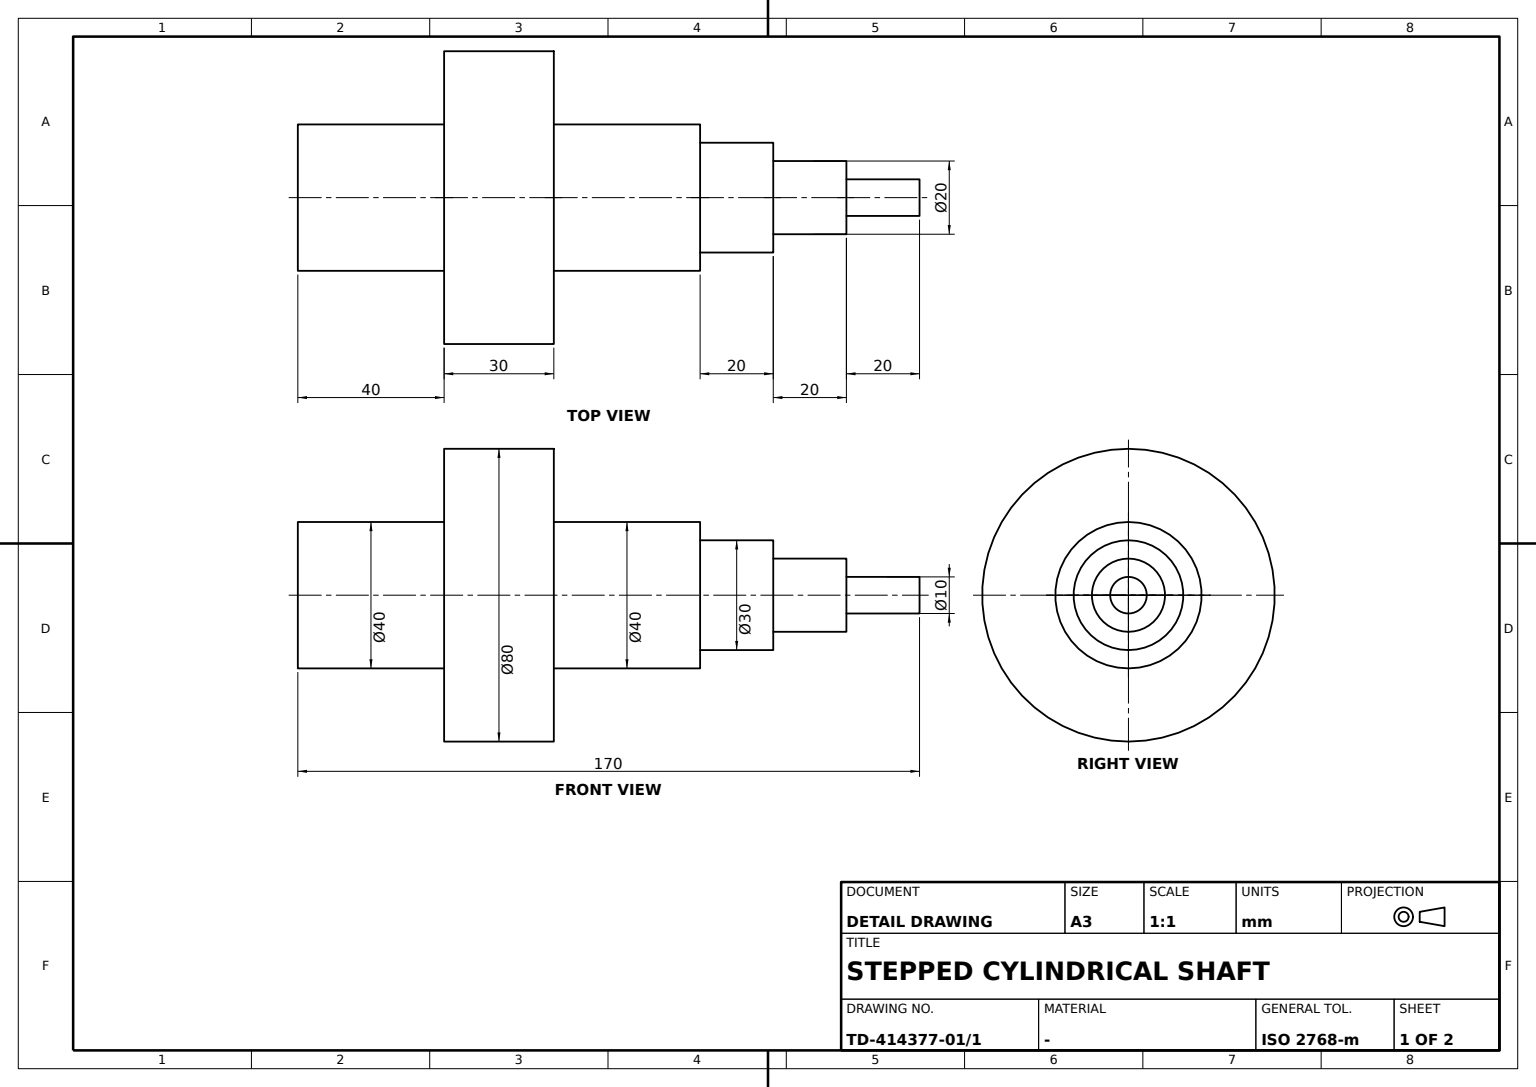
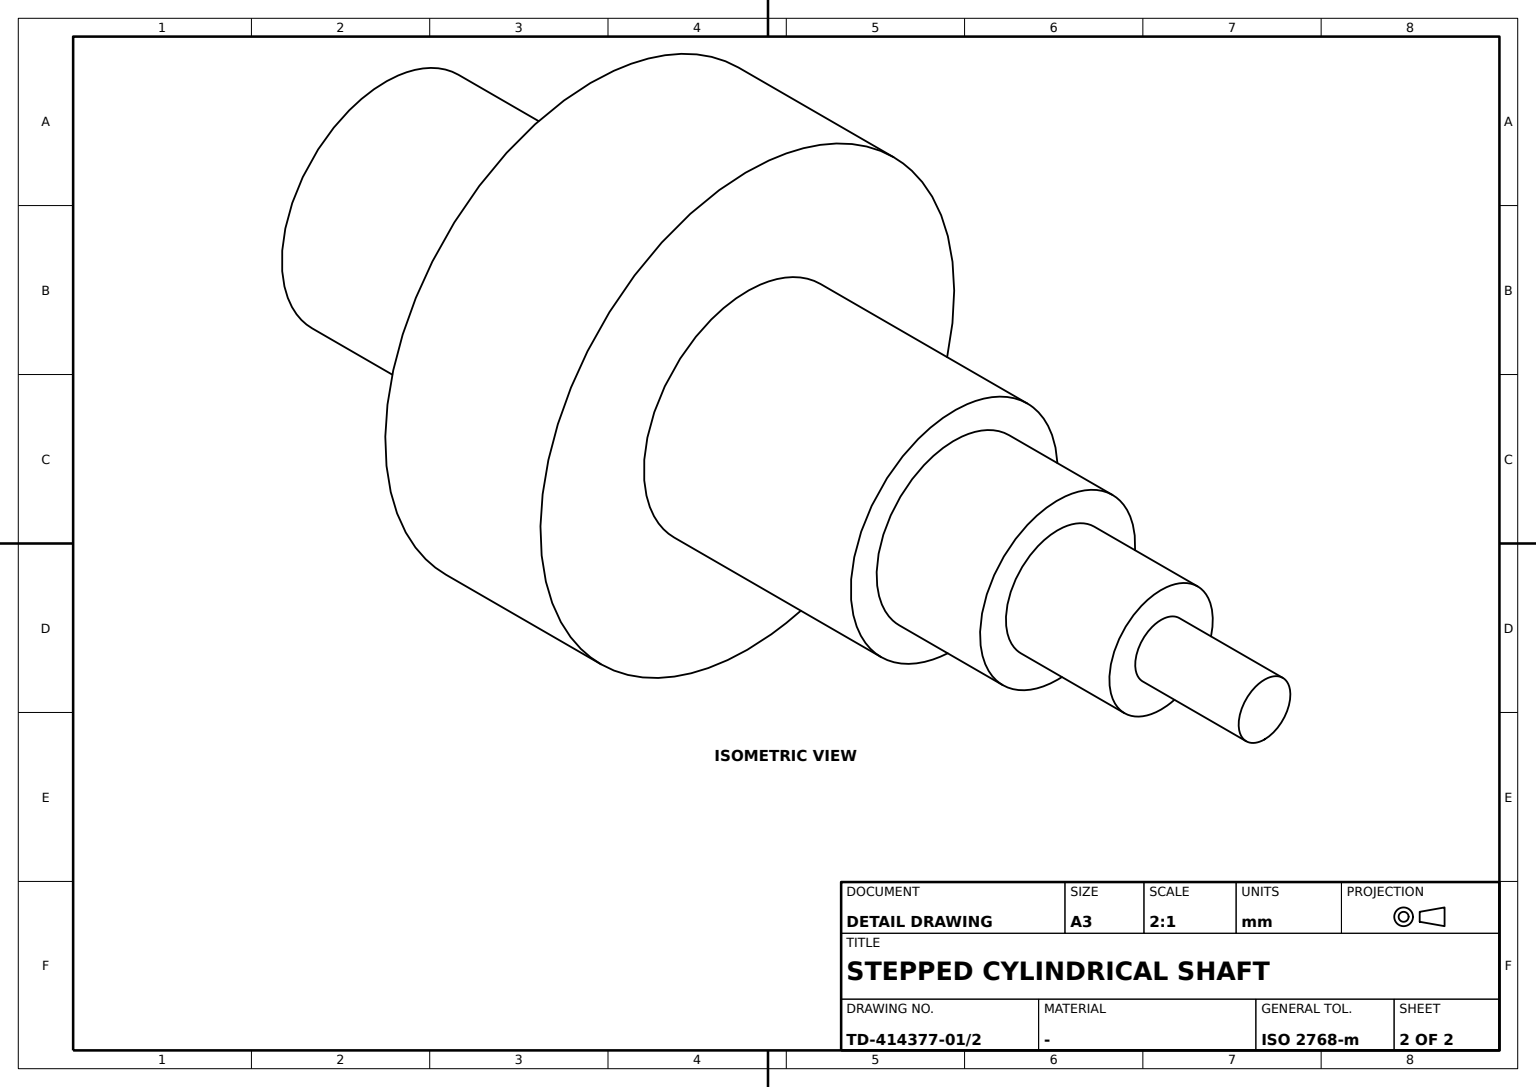
ISO-10303-21;
HEADER;
FILE_DESCRIPTION((''),'2;1');
FILE_NAME('','',(''),(''),'','','');
FILE_SCHEMA(('AUTOMOTIVE_DESIGN'));
ENDSEC;
DATA;
#1=APPLICATION_CONTEXT('');
#2=PRODUCT_CONTEXT('',#1,'mechanical');
#3=PRODUCT('','','',(#2));
#4=PRODUCT_DEFINITION_FORMATION('','',#3);
#5=PRODUCT_DEFINITION_CONTEXT('',#1,'design');
#6=PRODUCT_DEFINITION('','',#4,#5);
#7=PRODUCT_DEFINITION_SHAPE('','',#6);
#8=(LENGTH_UNIT()NAMED_UNIT(*)SI_UNIT(.MILLI.,.METRE.));
#9=(NAMED_UNIT(*)PLANE_ANGLE_UNIT()SI_UNIT($,.RADIAN.));
#10=(NAMED_UNIT(*)SI_UNIT($,.STERADIAN.)SOLID_ANGLE_UNIT());
#11=UNCERTAINTY_MEASURE_WITH_UNIT(LENGTH_MEASURE(0.005),#8,'distance_accuracy_value','');
#12=(GEOMETRIC_REPRESENTATION_CONTEXT(3)GLOBAL_UNCERTAINTY_ASSIGNED_CONTEXT((#11))GLOBAL_UNIT_ASSIGNED_CONTEXT((#8,#9,#10))REPRESENTATION_CONTEXT('',''));
#13=CARTESIAN_POINT('',(-42.006329,0.,-20.));
#14=VERTEX_POINT('',#13);
#15=CARTESIAN_POINT('',(-42.006329,0.,0.));
#16=DIRECTION('',(1.,0.,0.));
#17=DIRECTION('',(0.,0.,-1.));
#18=AXIS2_PLACEMENT_3D('',#15,#16,#17);
#19=CIRCLE('',#18,20.);
#20=EDGE_CURVE('',#14,#14,#19,.T.);
#21=ORIENTED_EDGE('',*,*,#20,.F.);
#22=EDGE_LOOP('',(#21));
#23=FACE_BOUND('',#22,.T.);
#24=CARTESIAN_POINT('',(-42.006329,0.,-40.));
#25=VERTEX_POINT('',#24);
#26=CIRCLE('',#18,40.);
#27=EDGE_CURVE('',#25,#25,#26,.T.);
#28=ORIENTED_EDGE('',*,*,#27,.T.);
#29=EDGE_LOOP('',(#28));
#30=FACE_BOUND('',#29,.T.);
#31=CARTESIAN_POINT('',(-42.006329,-40.,0.));
#32=DIRECTION('',(0.,1.,0.));
#33=AXIS2_PLACEMENT_3D('',#31,#16,#32);
#34=PLANE('',#33);
#35=ADVANCED_FACE('',(#23,#30),#34,.T.);
#36=CARTESIAN_POINT('',(-72.006329,0.,-20.));
#37=VERTEX_POINT('',#36);
#38=CARTESIAN_POINT('',(-72.006329,0.,0.));
#39=AXIS2_PLACEMENT_3D('',#38,#16,#17);
#40=CIRCLE('',#39,20.);
#41=EDGE_CURVE('',#37,#37,#40,.T.);
#42=ORIENTED_EDGE('',*,*,#41,.T.);
#43=EDGE_LOOP('',(#42));
#44=FACE_BOUND('',#43,.T.);
#45=CARTESIAN_POINT('',(-72.006329,0.,-40.));
#46=VERTEX_POINT('',#45);
#47=CIRCLE('',#39,40.);
#48=EDGE_CURVE('',#46,#46,#47,.T.);
#49=ORIENTED_EDGE('',*,*,#48,.F.);
#50=EDGE_LOOP('',(#49));
#51=FACE_BOUND('',#50,.T.);
#52=CARTESIAN_POINT('',(-72.006329,-20.,0.));
#53=AXIS2_PLACEMENT_3D('',#52,#16,#32);
#54=PLANE('',#53);
#55=ADVANCED_FACE('',(#44,#51),#54,.F.);
#56=CARTESIAN_POINT('',(17.993671,0.,-10.));
#57=VERTEX_POINT('',#56);
#58=CARTESIAN_POINT('',(17.993671,0.,0.));
#59=AXIS2_PLACEMENT_3D('',#58,#16,#17);
#60=CIRCLE('',#59,10.);
#61=EDGE_CURVE('',#57,#57,#60,.T.);
#62=ORIENTED_EDGE('',*,*,#61,.F.);
#63=EDGE_LOOP('',(#62));
#64=FACE_BOUND('',#63,.T.);
#65=CARTESIAN_POINT('',(17.993671,0.,-15.));
#66=VERTEX_POINT('',#65);
#67=CIRCLE('',#59,15.);
#68=EDGE_CURVE('',#66,#66,#67,.T.);
#69=ORIENTED_EDGE('',*,*,#68,.T.);
#70=EDGE_LOOP('',(#69));
#71=FACE_BOUND('',#70,.T.);
#72=CARTESIAN_POINT('',(17.993671,-15.,0.));
#73=AXIS2_PLACEMENT_3D('',#72,#16,#32);
#74=PLANE('',#73);
#75=ADVANCED_FACE('',(#64,#71),#74,.T.);
#76=ORIENTED_EDGE('',*,*,#41,.F.);
#77=EDGE_LOOP('',(#76));
#78=FACE_BOUND('',#77,.T.);
#79=CARTESIAN_POINT('',(-112.006329,0.,-20.));
#80=VERTEX_POINT('',#79);
#81=CARTESIAN_POINT('',(-112.006329,0.,0.));
#82=AXIS2_PLACEMENT_3D('',#81,#16,#17);
#83=CIRCLE('',#82,20.);
#84=EDGE_CURVE('',#80,#80,#83,.T.);
#85=ORIENTED_EDGE('',*,*,#84,.T.);
#86=EDGE_LOOP('',(#85));
#87=FACE_BOUND('',#86,.T.);
#88=CARTESIAN_POINT('',(-27.006329,0.,0.));
#89=AXIS2_PLACEMENT_3D('',#88,#16,#32);
#90=CYLINDRICAL_SURFACE('',#89,20.);
#91=ADVANCED_FACE('',(#78,#87),#90,.T.);
#92=CARTESIAN_POINT('',(57.993671,0.,-5.));
#93=VERTEX_POINT('',#92);
#94=CARTESIAN_POINT('',(57.993671,0.,0.));
#95=AXIS2_PLACEMENT_3D('',#94,#16,#17);
#96=CIRCLE('',#95,5.);
#97=EDGE_CURVE('',#93,#93,#96,.T.);
#98=ORIENTED_EDGE('',*,*,#97,.F.);
#99=EDGE_LOOP('',(#98));
#100=FACE_BOUND('',#99,.T.);
#101=CARTESIAN_POINT('',(37.993671,0.,-5.));
#102=VERTEX_POINT('',#101);
#103=CARTESIAN_POINT('',(37.993671,0.,0.));
#104=AXIS2_PLACEMENT_3D('',#103,#16,#17);
#105=CIRCLE('',#104,5.);
#106=EDGE_CURVE('',#102,#102,#105,.T.);
#107=ORIENTED_EDGE('',*,*,#106,.T.);
#108=EDGE_LOOP('',(#107));
#109=FACE_BOUND('',#108,.T.);
#110=CYLINDRICAL_SURFACE('',#89,5.);
#111=ADVANCED_FACE('',(#100,#109),#110,.T.);
#112=ORIENTED_EDGE('',*,*,#84,.F.);
#113=EDGE_LOOP('',(#112));
#114=FACE_BOUND('',#113,.T.);
#115=AXIS2_PLACEMENT_3D('',#81,#16,#32);
#116=PLANE('',#115);
#117=ADVANCED_FACE('',(#114),#116,.F.);
#118=ORIENTED_EDGE('',*,*,#97,.T.);
#119=EDGE_LOOP('',(#118));
#120=FACE_BOUND('',#119,.T.);
#121=CARTESIAN_POINT('',(57.993671,-5.,0.));
#122=AXIS2_PLACEMENT_3D('',#121,#16,#32);
#123=PLANE('',#122);
#124=ADVANCED_FACE('',(#120),#123,.T.);
#125=ORIENTED_EDGE('',*,*,#68,.F.);
#126=EDGE_LOOP('',(#125));
#127=FACE_BOUND('',#126,.T.);
#128=CARTESIAN_POINT('',(-2.006329,0.,-15.));
#129=VERTEX_POINT('',#128);
#130=CARTESIAN_POINT('',(-2.006329,0.,0.));
#131=AXIS2_PLACEMENT_3D('',#130,#16,#17);
#132=CIRCLE('',#131,15.);
#133=EDGE_CURVE('',#129,#129,#132,.T.);
#134=ORIENTED_EDGE('',*,*,#133,.T.);
#135=EDGE_LOOP('',(#134));
#136=FACE_BOUND('',#135,.T.);
#137=CYLINDRICAL_SURFACE('',#89,15.);
#138=ADVANCED_FACE('',(#127,#136),#137,.T.);
#139=CARTESIAN_POINT('',(-2.006329,0.,-20.));
#140=VERTEX_POINT('',#139);
#141=CIRCLE('',#131,20.);
#142=EDGE_CURVE('',#140,#140,#141,.T.);
#143=ORIENTED_EDGE('',*,*,#142,.F.);
#144=EDGE_LOOP('',(#143));
#145=FACE_BOUND('',#144,.T.);
#146=ORIENTED_EDGE('',*,*,#20,.T.);
#147=EDGE_LOOP('',(#146));
#148=FACE_BOUND('',#147,.T.);
#149=ADVANCED_FACE('',(#145,#148),#90,.T.);
#150=ORIENTED_EDGE('',*,*,#106,.F.);
#151=EDGE_LOOP('',(#150));
#152=FACE_BOUND('',#151,.T.);
#153=CARTESIAN_POINT('',(37.993671,0.,-10.));
#154=VERTEX_POINT('',#153);
#155=CIRCLE('',#104,10.);
#156=EDGE_CURVE('',#154,#154,#155,.T.);
#157=ORIENTED_EDGE('',*,*,#156,.T.);
#158=EDGE_LOOP('',(#157));
#159=FACE_BOUND('',#158,.T.);
#160=CARTESIAN_POINT('',(37.993671,-10.,0.));
#161=AXIS2_PLACEMENT_3D('',#160,#16,#32);
#162=PLANE('',#161);
#163=ADVANCED_FACE('',(#152,#159),#162,.T.);
#164=ORIENTED_EDGE('',*,*,#133,.F.);
#165=EDGE_LOOP('',(#164));
#166=FACE_BOUND('',#165,.T.);
#167=ORIENTED_EDGE('',*,*,#142,.T.);
#168=EDGE_LOOP('',(#167));
#169=FACE_BOUND('',#168,.T.);
#170=CARTESIAN_POINT('',(-2.006329,-20.,0.));
#171=AXIS2_PLACEMENT_3D('',#170,#16,#32);
#172=PLANE('',#171);
#173=ADVANCED_FACE('',(#166,#169),#172,.T.);
#174=ORIENTED_EDGE('',*,*,#48,.T.);
#175=EDGE_LOOP('',(#174));
#176=FACE_BOUND('',#175,.T.);
#177=ORIENTED_EDGE('',*,*,#27,.F.);
#178=EDGE_LOOP('',(#177));
#179=FACE_BOUND('',#178,.T.);
#180=CYLINDRICAL_SURFACE('',#89,40.);
#181=ADVANCED_FACE('',(#176,#179),#180,.T.);
#182=ORIENTED_EDGE('',*,*,#61,.T.);
#183=EDGE_LOOP('',(#182));
#184=FACE_BOUND('',#183,.T.);
#185=ORIENTED_EDGE('',*,*,#156,.F.);
#186=EDGE_LOOP('',(#185));
#187=FACE_BOUND('',#186,.T.);
#188=CYLINDRICAL_SURFACE('',#89,10.);
#189=ADVANCED_FACE('',(#184,#187),#188,.T.);
#190=CLOSED_SHELL('',(#35,#55,#75,#91,#111,#117,#124,#138,#149,#163,#173,#181,#189));
#191=MANIFOLD_SOLID_BREP('',#190);
#192=ADVANCED_BREP_SHAPE_REPRESENTATION('',(#191),#12);
#193=SHAPE_DEFINITION_REPRESENTATION(#7,#192);
ENDSEC;
END-ISO-10303-21;
